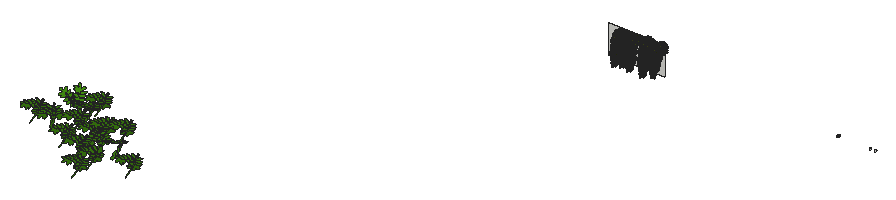
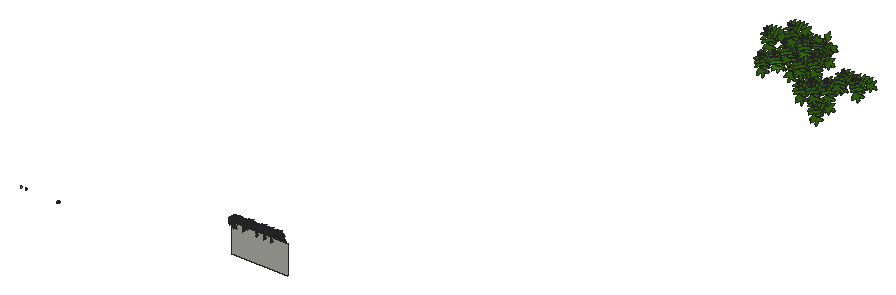
# SketchUp Ruby script. Lengths in inches.
U = 1.inch
M = Sketchup.active_model
def pt(a) = Geom::Point3d.new(a.map { |v| v * U })
def face(e, loops, mat)
  f = e.add_face(loops[0].map { |a| pt(a) })
  loops[1..].each { |l| e.add_face(l.map { |a| pt(a) }).erase! }
  f.material = f.back_material = mat if mat
  f
end
# faces: each face lists its corners as indices into pts; further lists are holes
def faces(e, pts, list, mat = nil) = list.each { |f| face(e, (f[0].is_a?(Array) ? f : [f]).map { |l| l.map { |i| pts[i] } }, mat) }
# xy, xz, yz: faces in a plane at the given z, y or x. An outline is a flat list of corners, or four numbers for a rectangle; further outlines are holes
def ring(l) = l.size == 4 ? [[l[0], l[1]], [l[2], l[1]], [l[2], l[3]], [l[0], l[3]]] : l.each_slice(2).to_a
def flat(e, list, mat, &to3) = list.each { |f| face(e, (f[0].is_a?(Array) ? f : [f]).map { |l| ring(l).map { |u, v| to3.(u, v) } }, mat) }
def xy(e, z, list, mat = nil) = flat(e, list, mat) { |x, y| [x, y, z] }
def xz(e, y, list, mat = nil) = flat(e, list, mat) { |x, z| [x, y, z] }
def yz(e, x, list, mat = nil) = flat(e, list, mat) { |y, z| [x, y, z] }
def lines(e, pts, list) = list.each { |a, b| e.add_line(pt(pts[a]), pt(pts[b])) }
# prism: a flat outline (further loops are holes) pulled along v
def prism(e, loops, v, mat = nil)
  f = face(e, loops, mat); d = Geom::Vector3d.new(v.map { |x| x * U })
  f.pushpull(f.normal.samedirection?(d) ? d.length : -d.length)
end
def box(e, o, s, mat = nil) = prism(e, [[o, [o[0] + s[0], o[1], o[2]], [o[0] + s[0], o[1] + s[1], o[2]], [o[0], o[1] + s[1], o[2]]]], [0, 0, s[2]], mat)
def at(x, y, z, deg = 0) = Geom::Transformation.translation(pt([x, y, z])) * Geom::Transformation.rotation(ORIGIN, Z_AXIS, deg.degrees)
def axes(o, x, y, z) = Geom::Transformation.new([*x, 0, *y, 0, *z, 0, *pt(o).to_a, 1])
def part(name) = M.definitions.add(name)
# library, detail: a bought-in or finely detailed component or shape, given as its bounding box
def library(name, o, s) = part(name).tap { |d| box(d.entities, o, s) }
def detail(e, o, s) = box(e.add_group.entities, o, s)
def put(e, d, t, mat = nil) = e.add_instance(d, t).tap { |i| i.material = mat if mat }
def group(e, t, mat = nil) = e.add_group.tap { |g| g.transformation = t; g.material = mat if mat }.entities
root = M.entities
M.materials.add("asdfasdfasdfasdf").color = [186, 198, 91]
M.materials.add("hojas").color = [70, 150, 19]
M.materials.add("leaf1_smaller_cleanasdfasfasdfas").color = [88, 95, 33]
M.materials.add("leaf2_smaller_cleansadfasdfasdfasd").color = [55, 66, 19]
c1 = part("rama-acacia")
p = [[-13.53,0.69,-1.07],[-13.38,0.86,-0.98],[-13.61,0.85,-1.06],[-14.07,0.85,-1.21],[-15.17,0.86,-1.58],[-15.95,0.92,-1.83],
  [-16.01,1,-1.83],[-16.01,1.17,-1.78],[-16.07,1.93,-1.6],[-16.4,2.73,-1.5],[-16.65,3.06,-1.5],[-17.13,4.01,-1.41],
  [-17.78,4.7,-1.44],[-18.28,5.07,-1.51],[-18.57,5.18,-1.58],[-18.91,5.47,-1.62],[-19.07,5.48,-1.67],[-19.35,5.61,-1.73],
  [-19.51,5.64,-1.78],[-19.38,5.57,-1.75],[-19.33,5.5,-1.75],[-19.31,5.23,-1.82],[-19.38,5.08,-1.89],[-19.41,4.84,-1.96],
  [-19.36,4.59,-2.01],[-19.43,4.55,-2.04],[-19.36,4.15,-2.125],[-19.21,3.7,-2.19],[-18.875,3.1,-2.24],[-18.61,2.78,-2.24],
  [-17.83,2.19,-2.13],[-17.4375,1.85,-2.09],[-17.04,1.49,-2.05],[-16.61,1.24,-1.97],[-16.17,1.0625,-1.87],[-16.06,0.95,-1.86],
  [-16.06,0.91,-1.87],[-16.32,0.9,-1.96],[-16.7,0.88,-2.1],[-17.05,0.91,-2.21],[-17.61,1.15,-2.33],[-18.06,1.29,-2.45],
  [-18.88,1.53,-2.67],[-20.25,1.46,-3.15],[-20.59,1.49,-3.26],[-20.79,1.37,-3.36],[-21.08,1.2,-3.5],[-21.28,1.22,-3.5625],
  [-21.48,0.94,-3.71],[-21.79,0.5,-3.93],[-22.02,0.17,-4.1],[-22.11,0.05,-4.16],[-22.21,-0.02,-4.21],[-22.375,-0.05,-4.28],
  [-22.375,-0.07,-4.28],[-22.18,-0.09,-4.22],[-22.11,-0.07,-4.19],[-21.78,-0.1,-4.09],[-21.6,-0.18,-4.05],[-21.52,-0.27,-4.04],
  [-21.33,-0.33,-4],[-20.94,-0.54,-3.92],[-20.6875,-0.63,-3.86],[-20.54,-0.68,-3.82],[-20.42,-0.67,-3.78],[-20.09,-0.46,-3.61],
  [-19.8,-0.24,-3.45],[-19.21,-0.02,-3.19],[-18.48,0.08,-2.92],[-17.72,0.38,-2.58],[-17.4,0.5,-2.4375],[-16.93,0.75,-2.21],
  [-16.78,0.8,-2.15],[-16.1,0.83,-1.91],[-16.0625,0.81,-1.9],[-16.08,0.77,-1.91],[-16.27,0.72,-1.99],[-16.88,0.39,-2.29],
  [-17.1875,0.15,-2.46],[-17.27,0.02,-2.52],[-17.94,-0.52,-2.89],[-17.94,-0.59,-2.91],[-18.08,-0.68,-2.99],[-18.13,-0.86,-3.05],
  [-18.56,-1.55,-3.38],[-18.71,-2.11,-3.58],[-18.79,-2.61,-3.74],[-18.86,-2.84,-3.83],[-18.87,-3.07,-3.89],[-18.84,-3.22,-3.92],
  [-18.8,-3.26,-3.92],[-18.76,-3.47,-3.96],[-18.76,-3.6,-4],[-18.67,-3.8,-4.02],[-18.61,-3.92,-4.04],[-18.58,-4.11,-4.07],
  [-18.53,-4.18,-4.08],[-18.58,-4.35,-4.14],[-18.65,-4.43,-4.18],[-18.72,-4.51,-4.23],[-18.8125,-4.51,-4.26],[-18.8125,-4.53,-4.26],
  [-18.72,-4.54,-4.24],[-18.66,-4.49,-4.21],[-18.58,-4.43,-4.16],[-18.35,-4.23,-4.03],[-18.32,-4.17,-4],[-18.22,-4.125,-3.95],
  [-18.1,-4,-3.88],[-17.79,-3.72,-3.7],[-17.68,-3.51,-3.61],[-17.32,-3.13,-3.38],[-17.24,-2.94,-3.31],[-16.78,-2.12,-2.93],
  [-16.48,-1.78,-2.73],[-16.3,-1.28,-2.54],[-16.05,-0.75,-2.3125],[-15.89,-0.2,-2.11],[-15.89,0.39,-1.95],[-15.96,0.79,-1.87],
  [-15.91,0.82,-1.84],[-15.27,0.8,-1.63],[-14.18,0.76,-1.27],[-13.78,0.73,-1.15],[-13.78,0.67,-1.16],[-14.23,0.54,-1.35],
  [-14.65,0.33,-1.55],[-14.97,0.02,-1.74],[-15.25,-0.36,-1.9375],[-15.57,-0.72,-2.14],[-15.96,-1.64,-2.52],[-16.2,-2.51,-2.84],
  [-16.2,-3.12,-3],[-16.14,-3.41,-3.06],[-16.1,-3.75,-3.14],[-16.1,-4.09,-3.23],[-16.2,-4.25,-3.3],[-16.2,-4.28,-3.3125],
  [-16.08,-4.19,-3.24],[-15.98,-4.08,-3.18],[-15.96,-3.94,-3.14],[-15.96,-3.8125,-3.1],[-15.9,-3.72,-3.06],[-15.68,-3.55,-2.9375],
  [-15.51,-3.49,-2.86],[-15.3,-3.33,-2.75],[-15.23,-3.17,-2.68],[-15.01,-3.03,-2.57],[-14.875,-2.83,-2.47],[-14.6,-2.59,-2.3125],
  [-14.4,-2.27,-2.16],[-14.12,-1.6,-1.89],[-13.91,-1.1,-1.68],[-13.67,-0.83,-1.53],[-13.53,-0.45,-1.38],[-13.53,0.67,-1.08],
  [-12.41,6.01,0.65],[-12.44,6.14,0.68],[-12.41,6.29,0.73],[-12.43,6.29,0.73],[-12.44,6.26,0.72],[-12.47,6.15,0.68],
  [-12.49,6.07,0.66],[-12.57,5.75,0.55],[-12.67,5.36,0.43],[-12.79,4.875,0.28],[-12.83,4.52,0.18],[-12.83,3.99,0.04],
  [-12.73,3.11,-0.18],[-12.58,2.52,-0.3125],[-12.3,1.97,-0.41],[-11.88,1.51,-0.46],[-11.37,1.0625,-0.48],[-10.75,0.75,-0.45],
  [-10.75,0.68,-0.47],[-12.55,0.7,-0.79],[-13.21,0.79,-0.89],[-13.2,0.67,-0.92],[-12.56,0.62,-0.82],[-11.15,0.56,-0.58],
  [-10.79,0.54,-0.52],[-10.72,0.52,-0.51],[-10.72,0.5,-0.52],[-10.87,0.47,-0.55],[-11.14,0.41,-0.62],[-11.39,0.27,-0.7],
  [-11.625,-0.01,-0.82],[-11.8,-0.43,-0.96],[-11.83,-0.57,-1],[-12.02,-1.08,-1.17],[-12.1,-1.39,-1.27],[-12.17,-1.95,-1.4375],
  [-12.17,-2.77,-1.65],[-12.09,-3.59,-1.86],[-11.86,-4.26,-2],[-11.8125,-4.4,-2.03],[-11.84,-4.49,-2.05],[-11.91,-4.6,-2.1],
  [-11.97,-4.65,-2.12],[-11.98,-4.67,-2.13],[-11.92,-4.65,-2.11],[-11.84,-4.59,-2.08],[-11.77,-4.52,-2.05],[-11.74,-4.47,-2.03],
  [-11.37,-4.3125,-1.92],[-10.95,-4.0625,-1.78],[-10.82,-3.89,-1.71],[-10.64,-3.57,-1.59],[-10.41,-3.05,-1.41],[-10.27,-2.73,-1.3],
  [-10.07,-1.88,-1.03],[-10.15,-0.71,-0.73],[-10.31,-0.1,-0.6],[-10.5,0.4,-0.5],[-10.5,0.48,-0.48],[-10.44,0.53,-0.45],
  [-10.39,0.64,-0.42],[-10.52,0.73,-0.42],[-10.44,0.93,-0.35],[-10.44,1.2,-0.28],[-10.32,1.47,-0.18],[-10.48,2.6875,0.12],
  [-10.43,2.96,0.2],[-10.75,3.87,0.38],[-11.26,4.93,0.57],[-11.8,5.54,0.64],[-12.37,5.93,0.64],[-7.78,0.19,-0.06],
  [-7.78,0.25,-0.04],[-7.75,0.39,0],[-7.89,0.4,-0.02],[-7.96,0.46,-0.02],[-7.96,0.49,-0.01],[-7.76,0.62,0.06],
  [-7.53,0.99,0.2],[-7.31,1.78,0.45],[-7.31,2.74,0.71],[-7.63,3.6875,0.9],[-8.02,4.57,1.07],[-8.66,5.23,1.13],
  [-8.83,5.4,1.14],[-8.92,5.54,1.16],[-9.1,5.64,1.16],[-9.08,5.6,1.15],[-9.02,5.56,1.15],[-8.94,5.46,1.14],
  [-8.9,5.37,1.12],[-8.9375,5.25,1.08],[-9.14,4.92,0.96],[-9.31,4.5625,0.83],[-9.39,3.73,0.6],[-9.44,2.76,0.32],
  [-9.23,1.59,0.05],[-8.82,0.9,-0.06],[-8.36,0.59,-0.0625],[-8.14,0.51,-0.04],[-8.05,0.48,-0.03],[-8.05,0.46,-0.04],
  [-8.12,0.43,-0.06],[-10.1,0.49,-0.4],[-8.22,0.3125,-0.11],[-8.22,0.25,-0.125],[-8.53,0.13,-0.21],[-8.8,-0.16,-0.34],
  [-8.96,-0.61,-0.49],[-8.96,-0.87,-0.56],[-9.16,-1.42,-0.74],[-9.13,-1.77,-0.83],[-9.09,-1.83,-0.84],[-9.125,-1.92,-0.87],
  [-9.125,-2.13,-0.93],[-9.08,-2.23,-0.95],[-9.15,-2.39,-1],[-9.11,-2.67,-1.07],[-9.03,-2.86,-1.11],[-9.07,-3.03,-1.16],
  [-8.97,-3.23,-1.19],[-8.93,-3.44,-1.24],[-8.93,-3.71,-1.32],[-8.79,-4.05,-1.38],[-8.7,-4.25,-1.42],[-8.7,-4.39,-1.46],
  [-8.76,-4.53,-1.5],[-8.77,-4.65,-1.54],[-8.64,-4.55,-1.49],[-8.27,-4.22,-1.33],[-8.1875,-4.06,-1.27],[-8.07,-3.98,-1.23],
  [-7.98,-3.79,-1.17],[-7.79,-3.59,-1.08],[-7.64,-3.3,-0.97],[-7.64,-3.25,-0.96],[-7.59,-3.21,-0.9375],[-7.52,-2.93,-0.85],
  [-7.52,-2.85,-0.83],[-7.47,-2.81,-0.81],[-7.3,-2.09,-0.59],[-7.32,-2.01,-0.57],[-7.27,-1.95,-0.54],[-7.1875,-1.57,-0.42],
  [-7.17,-1.46,-0.39],[-7.17,-1.16,-0.3125],[-7.23,-0.61,-0.17],[-7.49,-0.15,-0.1],[-13.39,-0.07,-1.23],[-13.39,0.25,-1.14],
  [-13.49,0.5625,-1.09],[-13.8,1.01,-1.08],[-13.61,0.91,-1.04],[-13.38,0.92,-0.96],[-13.32,1.03,-0.91],[-13.32,1.35,-0.82],
  [-13.28,1.49,-0.77],[-13.28,1.99,-0.64],[-13.44,2.67,-0.51],[-13.72,3.31,-0.43],[-13.93,3.71,-0.4],[-14.1,4.39,-0.27],
  [-14.5625,5.06,-0.25],[-14.89,5.62,-0.21],[-15.33,6.1,-0.23],[-15.65,6.8,-0.15],[-15.79,6.89,-0.18],[-15.61,6.52,-0.22],
  [-15.51,6.32,-0.24],[-15.45,6.28,-0.23],[-15.52,6,-0.32],[-15.63,5.6875,-0.45],[-15.77,4.97,-0.68],[-15.7,4.25,-0.85],
  [-15.46,3,-1.11],[-15,2.03,-1.21],[-14.3,1.29,-1.17],[-4.5625,0.33,0.09],[-4.22,0.49,0.13],[-4,0.7,0.1875],
  [-3.86,0.99,0.26],[-3.77,1.41,0.38],[-3.7,1.73,0.46],[-3.77,1.99,0.53],[-3.85,2.17,0.58],[-3.88,2.57,0.6875],
  [-3.98,2.9,0.78],[-4.0625,2.97,0.8],[-4.1,3.14,0.84],[-4.1875,3.25,0.87],[-4.27,3.55,0.95],[-4.31,3.71,0.99],
  [-4.42,3.9,1.04],[-4.625,4.2,1.125],[-4.72,4.39,1.18],[-4.89,4.57,1.23],[-4.98,4.73,1.27],[-5,4.72,1.26],
  [-5.01,4.51,1.21],[-4.96,4.32,1.16],[-4.97,4.27,1.14],[-5.14,3.78,1.01],[-5.3,3.39,0.91],[-5.44,2.76,0.74],
  [-5.5,2.09,0.56],[-5.57,1.78,0.48],[-5.57,1.42,0.38],[-5.57,1.09,0.29],[-5.47,0.72,0.19],[-5.22,0.44,0.12],
  [-4.93,0.27,0.07],[-4.76,0.22,0.06],[-4.76,0.18,0.05],[-4.83,0.16,0.04],[-5.26,0,0],[-5.34,-0.04,-0.01],
  [-5.47,-0.22,-0.06],[-5.51,-0.6,-0.16],[-5.42,-1.09,-0.29],[-5.28,-1.49,-0.4],[-5.21,-1.87,-0.5],[-5.11,-2.15,-0.57],
  [-5.08,-2.34,-0.63],[-5.01,-2.47,-0.66],[-4.96,-2.69,-0.72],[-4.86,-2.9375,-0.79],[-4.84,-3.07,-0.82],[-4.77,-3.18,-0.85],
  [-4.74,-3.43,-0.92],[-4.7,-3.71,-0.99],[-4.62,-3.89,-1.04],[-4.58,-3.98,-1.07],[-4.58,-3.83,-1.03],[-4.51,-3.67,-0.98],
  [-4.3,-3.32,-0.89],[-4.16,-3.09,-0.83],[-4.16,-2.98,-0.8],[-4.11,-2.92,-0.78],[-4.02,-2.8,-0.75],[-3.95,-2.59,-0.69],
  [-3.95,-2.33,-0.625],[-3.86,-2.26,-0.6],[-3.86,-2.02,-0.54],[-3.86,-1.44,-0.39],[-3.94,-1.22,-0.33],[-3.94,-1.08,-0.29],
  [-4,-0.96,-0.26],[-4,-0.87,-0.23],[-4.0625,-0.8125,-0.22],[-4.16,-0.54,-0.14],[-4.39,-0.24,-0.06],[-4.61,-0.08,-0.02],
  [-4.77,-0.03,-0.01],[-4.77,-0.01,0],[-4.65,-0.01,0],[-4.61,0.19,0.05],[-4.66,0.23,0.0625],[-4.63,0.29,0.08],
  [-4.07,0.17,0.04],[0,-0.24,-0.06],[0,0,0],[-0.5,0.04,0.01],[-1.58,0.08,0.02],[-13.78,0.67,-1.08]]
faces(c1.entities,p,[[0,1,2,3,4,5,6,7,8,9,10,11,12,13,14,15,16,17,18,19,20,21,22,23,24,25,26,27,28,29,30,31,32,33,34,35,36,37,38,39,40,41,42,43,44,45,46,47,48,49,50,51,52,53,54,55,56,57,58,59,60,61,62,63,64,65,66,67,68,69,70,71,72,73,74,75,76,77,78,79,80,81,82,83,84,85,86,87,88,89,90,91,92,93,94,95,96,97,98,99,100,101,102,103,104,105,106,107,108,109,110,111,112,113,114,115,116,117,118,119,120,121,122,123,124,125,126,127,128,129,130,131,132,133,134,135,136,137,138,139,140,141,142,143,144,145,146,147,148,149,150,151,152,153,154,155],[156,157,158,159,160,161,162,163,164,165,166,167,168,169,170,171,172,173,174,175,176,177,178,179,180,181,182,183,184,185,186,187,188,189,190,191,192,193,194,195,196,197,198,199,200,201,202,203,204,205,206,207,208,209,210,211,212,213,214,215,216,217,218,219,220,221,222,223,224,225,226],[227,228,229,230,231,232,233,234,235,236,237,238,239,240,241,242,243,244,245,246,247,248,249,250,251,252,253,254,255,256,257,258,216,215,259,260,261,262,263,264,265,266,267,268,269,270,271,272,273,274,275,276,277,278,279,280,281,282,283,284,285,286,287,288,289,290,291,292,293,294,295,296,297,298,299,300,301,302,303],[154,304,305,306,155],[307,308,1,309,310,311,312,313,314,315,316,317,318,319,320,321,322,323,324,325,326,327,328,329,330,331,332],[333,334,335,336,337,338,339,340,341,342,343,344,345,346,347,348,349,350,351,352,353,354,355,356,357,358,359,360,361,362,363,364,365,366,367,368,369,370,371,372,373,374,375,376,377,378,379,380,381,382,383,384,385,386,387,388,389,390,391,392,393,394,395,396,397,398,399,400,401,402,403,404,405,406,407,408,409,410,411,412,413],[0,177,1],[308,2,1],
  [176,1,177],[414,411,410,415,416,417,418],[228,370,229],[369,229,370]],"hojas")
lines(c1.entities,p,[[155,419]])
c2 = part("Group\#150")
put(c2.entities,c1,axes([10.13,10.27,0],[0.45315,0.21131,0],[-0.21131,0.45315,0],[0,0,0.5]))
put(c2.entities,c1,axes([10.13,10.27,0],[0.11638,0.47539,0.10227],[-0.48087,0.12813,-0.0484],[-0.07223,-0.08709,0.48703]))
put(c2.entities,c1,axes([9.58,10.26,-0.7],[0.1449,0.38901,-0.2787],[-0.10883,0.31035,0.37662],[0.46601,-0.04848,0.17461]))
c3 = part("Group\#151")
put(c3.entities,c2,axes([24.99,4.24,9.59],[0.78856,0.61496,0],[0.01473,-0.01889,0.99971],[0.61478,-0.78833,-0.02396]))
put(c3.entities,c2,axes([39.5,6.625,12.55],[0.6544,0.49291,0.57341],[-0.44023,-0.3682,0.81892],[0.61478,-0.78833,-0.02396]))
put(c3.entities,c2,axes([32.34,3.7,6.88],[0.78856,0.61496,0],[0.01473,-0.01889,0.99971],[0.61478,-0.78833,-0.02396]))
put(c3.entities,c2,axes([43.14,6.65,17.54],[0.78856,0.61496,0],[0.35273,-0.4523,0.81915],[0.50374,-0.64595,-0.57358]))
put(c3.entities,c2,axes([12.2,6.2,16.68],[0.7209,0.54936,0.4225],[-0.31991,-0.27701,0.90605],[0.61478,-0.78833,-0.02396]))
put(c3.entities,c2,axes([49.9375,3.79,26.09],[0.78856,0.61496,0],[0.01473,-0.01889,0.99971],[0.61478,-0.78833,-0.02396]))
put(c3.entities,c2,axes([36.11,4.9375,33.94],[0.78856,0.61496,0],[0.01473,-0.01889,0.99971],[0.61478,-0.78833,-0.02396]))
put(c3.entities,c2,axes([39.61,3.79,23.47],[0.78856,0.61496,0],[0.01473,-0.01889,0.99971],[0.61478,-0.78833,-0.02396]))
put(c3.entities,c2,axes([25.59,6.5625,46.47],[-0.40704,-0.29112,-0.86578],[0.67555,0.54201,-0.49986],[0.61478,-0.78833,-0.02396]))
put(c3.entities,c2,axes([54.97,1.98,11.65],[0.78856,0.61496,0],[0.01473,-0.01889,0.99971],[0.61478,-0.78833,-0.02396]))
put(c3.entities,c2,axes([32.97,3.79,19.14],[0.78856,0.61496,0],[0.01473,-0.01889,0.99971],[0.61478,-0.78833,-0.02396]))
put(c3.entities,c2,axes([24.24,3.79,21.99],[0.78856,0.61496,0],[0.01473,-0.01889,0.99971],[0.61478,-0.78833,-0.02396]))
put(c3.entities,c2,axes([16.86,4.24,12.3],[0.78856,0.61496,0],[0.01473,-0.01889,0.99971],[0.61478,-0.78833,-0.02396]))
put(c3.entities,c2,axes([1.23,3.9375,19.07],[0.78856,0.61496,0],[0.01473,-0.01889,0.99971],[0.61478,-0.78833,-0.02396]))
put(c3.entities,c2,axes([29.05,5.25,29.11],[0.78856,0.61496,0],[0.21033,-0.2697,0.93969],[0.57787,-0.741,-0.34202]))
put(c3.entities,c2,axes([24.16,3.79,-0.1],[0.78856,0.61496,0],[0.01473,-0.01889,0.99971],[0.61478,-0.78833,-0.02396]))
c4 = part("leaf1a")
p = [[1.06,3.74,11.78],[8.28,8.7,-0.64],[9.51,5.4,26.1],[17.76,4.04,11.26],[17.85,2.23,20],[14.31,3.29,26.73],
  [3.78,3.8125,25.98],[-0.21,2.38,19.72]]
faces(c4.entities,p,[[0,1,2],[2,1,3],[3,4,5],[3,5,2],[6,7,0],[0,2,6]],"leaf1_smaller_cleanasdfasfasdfas")
c5 = part("leaf2a")
p = [[1.4375,3.56,10.81],[8.71,6.8,-0.73],[9.51,3.5,26.59],[16.66,3.91,9.8],[17.86,1.3,19.21],[14.9,1.58,24.92],
  [5.15,2.55,24.01],[1.29,1.87,19.875]]
faces(c5.entities,p,[[0,1,2],[2,1,3],[3,4,5],[3,5,2],[6,7,0],[0,2,6]],"leaf2_smaller_cleansadfasdfasdfasd")
c6 = part("Group\#220")
put(c6.entities,c5,axes([6.68,1.92,2.42],[-0.04671,0.11082,0.08136],[0.07715,0.09226,-0.08136],[-0.11379,0.01705,-0.08856]))
put(c6.entities,c4,axes([1.26,0.54,1.25],[0.13756,-0.04533,0.01029],[0.0079,-0.00888,-0.14471],[0.04581,0.13766,-0.00594]))
put(c6.entities,c5,axes([-0.51,4.89,1.49],[-0.00057,-0.14139,-0.03304],[0.00922,0.03294,-0.14111],[0.14491,-0.00265,0.00885]))
put(c6.entities,c4,axes([4.37,7.98,1.26],[-0.14226,-0.02905,0],[0,0,-0.1452],[0.02905,-0.14226,0]))
put(c6.entities,c4,axes([1.46,4.03,4.07],[0.06242,-0.12847,-0.02614],[-0.10319,-0.03029,-0.09755],[0.08086,0.06051,-0.10432]))
c7 = part("leaf_a")
p = [[1.43,4.41,0.74],[1.39,4.36,0.69],[1.39,4.61,0.21],[1.43,4.67,0.24],[1.35,4.41,0.74],[1.35,4.67,0.24],
  [1.35,3.9,1.02],[1.43,3.9,1.02],[1.39,3.89,0.95],[1.39,3.35,0.9],[1.43,3.34,0.96],[1.35,3.34,0.96]]
faces(c7.entities,p,[[0,1,2,3],[1,4,5,2],[4,0,3,5],[3,2,5],[6,7,0,4],[8,6,4,1],[7,8,1,0],[9,10,11],
  [9,11,6,8],[10,9,8,7],[11,10,7,6]],"asdfasdfasdfasdf")
put(c7.entities,c5,axes([0,-0.08,0.875],[0.1452,0,0],[0,0.02746,-0.14258],[0,0.14258,0.02746]))
c8 = part("leaf_b")
prism(c8.entities,[[[1.36,4.21,-0.25],[1.31,4.13,-0.29],[1.26,4.21,-0.25]]],[0,-0.66,1.14],"asdfasdfasdfasdf")
put(c8.entities,c4,axes([0,-0.1,0.68],[0.1452,-0.0002,0],[0.00006,0.04124,-0.13922],[0.00019,0.13922,0.04124]))
c9 = part("Group\#209")
p = [[2.87,4.13,4.15],[2.98,3.98,4.12],[2.98,4.66,2.59],[2.87,4.8,2.65],[3.09,4.13,4.15],[3.09,4.8,2.65],
  [2.87,4.13,6.07],[2.98,3.98,6.12],[3.09,4.13,6.07],[2.87,5.04,7.34],[2.98,4.91,7.43],[3.09,5.04,7.34]]
faces(c9.entities,p,[[0,1,2,3],[1,4,5,2],[6,7,1,0],[7,8,4,1],[9,10,7,6],[10,11,8,7]],"asdfasdfasdfasdf")
put(c9.entities,c7,axes([0.86,0.51,1.53],[0.95176,-0.27809,0.12967],[0.18405,0.85554,0.48392],[-0.24551,-0.43671,0.86545]))
put(c9.entities,c8,axes([-0.97,2.96,6.52],[0.70711,-0.61237,-0.35355],[0.70711,0.61237,0.35355],[0,-0.5,0.86603]))
put(c9.entities,c7,axes([3.23,0.39,0.41],[0.82736,0.50176,-0.25242],[-0.32519,0.79434,0.5131],[0.45796,-0.34244,0.82037]))
put(c9.entities,c7,axes([3.25,-0.58,4.78],[0.8251,0.44069,-0.35355],[-0.31829,0.8796,0.35355],[0.46679,-0.17918,0.86603]))
c10 = part("Group\#2")
p = [[1.22,4.71,2.14],[1.31,4.57,2.14],[2.16,4.71,3.79],[2.24,4.57,3.77],[1.39,4.71,2.14],[2.33,4.71,3.79],
  [1.93,3.51,6.2],[1.85,3.64,6.23],[2.02,3.64,6.23],[0.93,3.38,8.58],[0.85,3.52,8.58],[1.02,3.52,8.58],
  [0.81,3.57,10.77],[0.72,3.71,10.73],[0.89,3.71,10.73],[1.31,4.57,13.2],[1.22,4.7,13.15],[1.39,4.7,13.15]]
faces(c10.entities,p,[[0,1,2],[3,2,1],[1,4,3],[5,3,4],[6,7,3],[6,3,8],[2,3,7],[5,8,3],
  [9,10,6],[9,6,11],[7,6,10],[8,11,6],[9,11,12],[9,12,10],[13,10,12],[14,12,11],
  [12,15,13],[12,14,15],[16,13,15],[17,15,14]],"asdfasdfasdfasdf")
put(c10.entities,c8,axes([3.93,1.17,1.97],[0.75139,0.49793,0.43299],[-0.65983,0.56085,0.50006],[0.00615,-0.66145,0.74997]))
put(c10.entities,c8,axes([6.23,5.09,1.92],[-0.36585,0.92196,0.12706],[-0.79398,-0.38042,0.47421],[0.48554,0.0726,0.87119]))
put(c10.entities,c8,axes([0.03,0.92,11.26],[1,0,0],[0,0.86603,0.5],[0,-0.5,0.86603]))
put(c10.entities,c7,axes([4.37,2.0625,9.11],[0.45529,0.76896,0.44879],[-0.86129,0.25267,0.44084],[0.22559,-0.58725,0.77733]))
put(c10.entities,c7,axes([1.89,-0.25,4.42],[0.88717,0.14116,0.43931],[-0.36372,0.79981,0.47751],[-0.28396,-0.58342,0.76091]))
put(c10.entities,c7,axes([-0.4,-0.0625,7.9],[0.80178,0.42258,-0.42258],[0,0.70711,0.70711],[0.59763,-0.56694,0.56694]))
put(c10.entities,c8,axes([0.05,0.6875,0.65],[0.97178,0.10445,-0.21151],[0.0126,0.87237,0.48869],[0.23556,-0.47756,0.84643]))
put(c10.entities,c7,axes([5.56,1.19,4.08],[0.24789,0.96746,-0.05068],[-0.86286,0.24427,0.4425],[0.44048,-0.06596,0.89533]))
put(c10.entities,c8,axes([4.91,2.14,7.29],[-0.04249,0.96546,-0.25705],[-0.89911,0.07524,0.4312],[0.43565,0.24944,0.86486]))
c11 = part("Group\#208")
put(c11.entities,c5,axes([5.59,5.52,3.3],[-0.07606,0.12201,-0.02028],[0.09645,0.0436,-0.0994],[-0.07744,-0.06554,-0.10388]))
put(c11.entities,c5,axes([7.69,4.27,1.08],[-0.09839,0.10661,0.00609],[-0.00698,0.00184,-0.14502],[-0.10656,-0.09856,0.00388]))
put(c11.entities,c4,axes([3.51,6.9,2.1],[-0.1403,-0.03711,-0.00465],[-0.00046,0.01976,-0.14385],[0.03739,-0.13898,-0.01921]))
put(c11.entities,c5,axes([2.18,0.07,1.375],[0.14025,0.00096,-0.03757],[-0.03758,0.00358,-0.14021],[0,0.14515,0.00371]))
put(c11.entities,c4,axes([-0.62,2,1.16],[0.081,-0.0806,-0.00996],[0.00004,0.01411,-0.11384],[0.08122,0.08039,0.00999]))
c12 = part("Group\#221")
p = [[1.22,4.71,2.14],[1.31,4.57,2.14],[2.16,4.71,3.79],[2.24,4.57,3.77],[1.39,4.71,2.14],[2.33,4.71,3.79],
  [1.93,3.51,6.2],[1.85,3.64,6.23],[2.02,3.64,6.23],[0.93,3.38,8.58],[0.85,3.52,8.58],[1.02,3.52,8.58],
  [0.81,3.57,10.77],[0.72,3.71,10.73],[0.89,3.71,10.73],[1.31,4.57,13.2],[1.22,4.7,13.15],[1.39,4.7,13.15]]
faces(c12.entities,p,[[0,1,2],[3,2,1],[1,4,3],[5,3,4],[6,7,3],[6,3,8],[2,3,7],[5,8,3],
  [9,10,6],[9,6,11],[7,6,10],[8,11,6],[9,11,12],[9,12,10],[13,10,12],[14,12,11],
  [12,15,13],[12,14,15],[16,13,15],[17,15,14]],"asdfasdfasdfasdf")
put(c12.entities,c8,axes([3.93,1.17,1.97],[0.75139,0.49793,0.43299],[-0.65983,0.56085,0.50006],[0.00615,-0.66145,0.74997]))
put(c12.entities,c8,axes([6.23,5.09,1.92],[-0.36585,0.92196,0.12706],[-0.79398,-0.38042,0.47421],[0.48554,0.0726,0.87119]))
put(c12.entities,c8,axes([0.03,0.92,11.26],[1,0,0],[0,0.86603,0.5],[0,-0.5,0.86603]))
put(c12.entities,c7,axes([4.37,2.0625,9.11],[0.45529,0.76896,0.44879],[-0.86129,0.25267,0.44084],[0.22559,-0.58725,0.77733]))
put(c12.entities,c7,axes([1.89,-0.25,4.42],[0.88717,0.14116,0.43931],[-0.36372,0.79981,0.47751],[-0.28396,-0.58342,0.76091]))
put(c12.entities,c7,axes([-0.4,-0.0625,7.9],[0.80178,0.42258,-0.42258],[0,0.70711,0.70711],[0.59763,-0.56694,0.56694]))
put(c12.entities,c8,axes([0.05,0.6875,0.65],[0.97178,0.10445,-0.21151],[0.0126,0.87237,0.48869],[0.23556,-0.47756,0.84643]))
put(c12.entities,c7,axes([5.56,1.19,4.08],[0.24789,0.96746,-0.05068],[-0.86286,0.24427,0.4425],[0.44048,-0.06596,0.89533]))
put(c12.entities,c8,axes([4.91,2.14,7.29],[-0.04249,0.96546,-0.25705],[-0.89911,0.07524,0.4312],[0.43565,0.24944,0.86486]))
c13 = part("Trailing philodendron")
put(c13.entities,c4,axes([3.65,12.52,19.68],[-0.0527,-0.13492,0.0101],[-0.03487,0.00307,-0.14092],[0.13073,-0.05357,-0.03351]))
put(c13.entities,c4,axes([5.13,11.34,20.6],[-0.03432,-0.12484,0.06572],[-0.08608,-0.03507,-0.11155],[0.11179,-0.06533,-0.06572]))
put(c13.entities,c5,axes([2.61,13.04,18.63],[0.05838,-0.12752,0.03758],[0.01564,-0.03417,-0.14025],[0.13202,0.06044,0]))
put(c13.entities,c5,axes([3.7,9.83,20.73],[-0.00129,-0.14519,0],[-0.0726,0.00064,-0.12575],[0.12574,-0.00112,-0.0726]))
put(c13.entities,c5,axes([11.375,11.11,20.23],[-0.14171,0.00126,0.03163],[-0.02867,0.05638,-0.1307],[-0.01341,-0.1338,-0.05478]))
put(c13.entities,c4,axes([2.4375,12.45,15.12],[-0.02375,-0.14324,0],[0.13106,-0.02173,-0.05859],[0.05781,-0.00958,0.13285]))
put(c13.entities,c4,axes([9.62,10.68,22.01],[0.05693,0.12487,-0.04742],[0.05061,-0.06787,-0.11796],[-0.12361,0.02972,-0.07014]))
put(c13.entities,c4,axes([11.63,16.35,20.5625],[-0.12691,-0.00762,0.07014],[-0.06947,0.03872,-0.12148],[-0.01233,-0.13973,-0.03749]))
put(c13.entities,c4,axes([12.51,17.52,17.81],[-0.1445,0.01001,0.0102],[-0.01383,-0.07182,-0.12544],[-0.0036,-0.1258,0.07242]))
put(c13.entities,c5,axes([9.09,6.34,22.72],[-0.09269,-0.05068,-0.09962],[-0.03661,0.13604,-0.03515],[0.1056,0.00268,-0.09962]))
put(c13.entities,c4,axes([4.83,12.62,22.54],[0.10783,0.09684,-0.00888],[0.09716,-0.10783,0.00397],[-0.00394,-0.00889,-0.14487]))
put(c13.entities,c4,axes([4.94,9.48,20.375],[0.01323,0.07633,0.07653],[0.10803,-0.00667,-0.01203],[-0.00375,0.07738,-0.07653]))
put(c13.entities,c5,axes([14,13.64,21.84],[-0.01852,-0.13907,0.03741],[-0.14373,0.01547,-0.01367],[0.00911,-0.03878,-0.13963]))
put(c13.entities,c5,axes([9.23,4.15,18.71],[0.14198,0.00177,-0.03038],[-0.02867,0.05638,-0.1307],[0.01021,0.13379,0.05548]))
put(c13.entities,c5,axes([5.82,4.5625,15.3],[0.13095,-0.05433,0.03137],[0.06268,0.11013,-0.07089],[0.00273,0.07747,0.12278]))
put(c13.entities,c6,axes([6.59,5.29,16.06],[1.23201,0.26412,0],[-0.26412,1.23201,0],[0,0,1.26]))
put(c13.entities,c9,axes([12.21,1.69,0.66],[-0.82914,0.03045,-0.02227],[0.02366,0.80139,0.21474],[-0.02938,-0.21389,0.80143]))
put(c13.entities,c10,axes([6.8125,1.15,7.57],[0.74375,-0.41052,0.02847],[0.41052,0.73612,-0.11],[0.02847,0.11,0.84237]))
put(c13.entities,c9,axes([-1.68,6.875,13.2],[0.5,-0.86603,0],[0.81585,0.47103,-0.33545],[0.29051,0.16773,0.94206]))
put(c13.entities,c9,axes([1.86,19.56,12.8125],[0.88164,0.4704,0.03781],[0.46333,-0.8476,-0.25863],[0.08962,-0.24554,0.96524]))
g1 = group(c13.entities,at(9.13,11.13,20.67))
put(g1,c5,axes([7.36,4.03,-0.3],[-0.05057,0.11966,-0.06487],[0.07036,-0.03625,-0.12173],[-0.11651,-0.07383,-0.04536]))
put(g1,c5,axes([8.4,1.56,-2.35],[-0.06703,0.12496,-0.03122],[-0.04831,-0.05702,-0.12449],[-0.1194,-0.04708,0.0679]))
put(g1,c4,axes([5.37,5.58,-2.1],[-0.14013,0.0124,0.03596],[-0.03803,-0.04347,-0.13322],[-0.00061,-0.13798,0.0452]))
put(g1,c5,axes([2.45,-0.07,0.8],[0.12002,-0.06072,-0.05468],[-0.07506,-0.04353,-0.11642],[0.03229,0.1245,-0.06737]))
put(g1,c4,axes([0.19,2.38,0.125],[0.05529,-0.09889,0.01797],[-0.03005,-0.03583,-0.10474],[0.09591,0.04578,-0.04318]))
put(c13.entities,c11,axes([17.33,10.54,16.15],[-0.62797,0.46654,0.62289],[-0.59637,-0.80271,0],[0.5,-0.37147,0.78231]))
put(c13.entities,c6,axes([3.44,11.88,17.73],[0.78616,-0.36326,0.5],[0.52263,0.82256,-0.22414],[-0.32986,0.43753,0.83652]))
put(c13.entities,c11,axes([5.5,5.07,16.54],[0.96593,-0.11102,0.2338],[0,0.90334,0.42894],[-0.25882,-0.41432,0.87255]))
put(c13.entities,c9,axes([18.84,3.62,12.91],[-0.80696,-0.59061,0],[-0.57048,0.77946,-0.25882],[-0.15286,0.20886,0.96593]))
put(c13.entities,c10,axes([3.89,0.96,5.21],[0.83948,0.00528,-0.02906],[-0.009,0.83292,-0.10846],[0.02813,0.1087,0.83246]))
put(c13.entities,c10,axes([6.1,0.84,-5.33],[0.875,-0.48296,0.03349],[0.48296,0.86603,-0.12941],[0.03349,0.12941,0.99103]))
put(c13.entities,c10,axes([3.87,-0.55,-8.84],[0.99938,0.00629,-0.0346],[-0.01071,0.99157,-0.12912],[0.03349,0.12941,0.99103]))
put(c13.entities,c9,axes([0.46,6.875,13.01],[0.5,-0.86603,0],[0.81585,0.47103,-0.33545],[0.29051,0.16773,0.94206]))
put(c13.entities,c10,axes([10.39,0.84,1.73],[0.875,-0.48296,0.03349],[0.48296,0.86603,-0.12941],[0.03349,0.12941,0.99103]))
put(c13.entities,c10,axes([-0.75,1.13,2.67],[0.7525,-0.41535,0.0288],[0.41535,0.74478,-0.11129],[0.0288,0.11129,0.85228]))
put(c13.entities,c10,axes([0.04,-0.97,-8.67],[0.735,-0.40569,0.02813],[0.40569,0.72746,-0.1087],[0.02813,0.1087,0.83246]))
put(c13.entities,c10,axes([0.09,-0.6,-7.42],[0.47403,-0.32078,-0.33698],[0.20171,0.57521,-0.26383],[0.41925,0.08595,0.50794]))
put(c13.entities,c10,axes([10.35,0.97,-6.0625],[0.76125,-0.42018,0.02914],[0.42018,0.75344,-0.11259],[0.02914,0.11259,0.86219]))
put(c13.entities,c10,axes([10.78,-1.55,-11.77],[0.72777,-0.42018,0.22517],[0.435,0.75344,0],[-0.19501,0.11259,0.84036]))
put(c13.entities,c10,axes([5.78,-1.55,-20.23],[0.76125,-0.42018,0.02914],[0.42018,0.75344,-0.11259],[0.02914,0.11259,0.86219]))
put(c13.entities,c10,axes([8.72,-1.43,-13.97],[0.65467,-0.36135,0.02506],[0.36135,0.64796,-0.09682],[0.02506,0.09682,0.74149]))
put(c13.entities,c12,axes([1.53,-0.97,-19.86],[0.735,-0.40569,0.02813],[0.40569,0.72746,-0.1087],[0.02813,0.1087,0.83246]))
put(c13.entities,c12,axes([6.23,-2.02,-7.18],[0.55125,-0.30427,0.0211],[0.39555,0.70927,-0.10599],[0.0211,0.08153,0.62435]))
put(c13.entities,c12,axes([6.43,-1.89,6.18],[0.735,-0.40569,0.02813],[0.5274,0.9457,-0.14132],[0.02813,0.1087,0.83246]))
put(c13.entities,c12,axes([10.24,1.09,9.64],[0.62475,-0.34484,0.02391],[0.44829,0.80384,-0.12012],[0.02391,0.0924,0.70759]))
put(c13.entities,c9,axes([1.56,7.74,12.8125],[-0.22619,0.97335,0.03781],[0.93864,0.22817,-0.25863],[0.26037,0.02301,0.96524]))
put(c13.entities,c9,axes([0.65,14.36,12.8125],[0.30411,0.95189,0.03781],[0.92309,-0.28464,-0.25863],[0.23543,-0.11355,0.96524]))
put(c13.entities,c9,axes([7.75,10.38,12.8125],[-0.84074,0.54011,0.03781],[0.51385,0.81797,-0.25863],[0.17062,0.19802,0.96524]))
put(c13.entities,c9,axes([12.92,19.16,12.8125],[0.9234,-0.38197,0.03781],[-0.36017,-0.89632,-0.25863],[-0.13268,-0.22521,0.96524]))
put(c13.entities,c9,axes([6.55,17.22,12.8125],[0.7985,0.60081,0.03781],[0.58857,-0.76596,-0.25863],[0.12643,-0.22877,0.96524]))
put(c13.entities,c9,axes([16.24,8.94,12.8125],[-0.64953,-0.75939,0.03781],[-0.7404,0.62041,-0.25863],[-0.17295,0.19599,0.96524]))
put(c13.entities,c9,axes([15.6875,15.74,12.8125],[0.12972,-0.99083,0.03781],[-0.95648,-0.13509,-0.25863],[-0.26137,0.00261,0.96524]))
put(c13.entities,c9,axes([19.85,8,15.61],[-0.64953,-0.75939,0.03781],[-0.7404,0.62041,-0.25863],[-0.17295,0.19599,0.96524]))
put(c13.entities,c9,axes([18.86,17.5,12.8125],[0.62831,-0.77705,0.03781],[-0.74495,-0.61494,-0.25863],[-0.22422,-0.13434,0.96524]))
put(c13.entities,c9,axes([-0.43,13.28,13.2],[-0.41945,-0.90778,0],[0.85518,-0.39515,-0.33545],[0.30452,-0.14071,0.94206]))
put(c13.entities,c12,axes([4.5625,-2.01,7.45],[0.56595,-0.31238,0.02166],[0.40609,0.72819,-0.10881],[0.02166,0.0837,0.641]))
put(c13.entities,c12,axes([4.48,-2.02,-24.24],[0.55125,-0.30427,0.0211],[0.39555,0.70927,-0.10599],[0.0211,0.08153,0.62435]))
put(c13.entities,c12,axes([4.9,-4.23,-11.04],[0.55125,-0.30427,0.0211],[0.39555,0.70927,-0.10599],[0.0211,0.08153,0.62435]))
put(c13.entities,c11,axes([17.33,10.54,17.41],[-0.62797,0.46654,0.62289],[-0.59637,-0.80271,0],[0.5,-0.37147,0.78231]))
put(c13.entities,c9,axes([-0.03,6.82,20.63],[0.44714,-0.87214,-0.19857],[0.53417,0.43844,-0.7228],[0.71744,0.21712,0.66191]))
put(c13.entities,c9,axes([20.82,12.8,12.8125],[0.12972,-0.99083,0.03781],[-0.95648,-0.13509,-0.25863],[-0.26137,0.00261,0.96524]))
xz(root,776.37,[[3153.83,138.1875,3240.72,183.3125]])
xz(root,799.91,[[3492.44,131.88,3492.73,131.92,3493,132.03,3493.24,132.21,3493.41,132.44,3493.53,132.71,3493.57,133,3493.53,133.29,3493.41,133.57,3493.24,133.8,3493,133.98,3492.73,134.09,3492.44,134.13,3492.15,134.09,3491.88,133.98,3491.65,133.8,3491.47,133.57,3491.35,133.29,3491.32,133,3491.35,132.71,3491.47,132.44,3491.65,132.21,3491.88,132.03,3492.15,131.92],[3543.57,131.88,3543.86,131.92,3544.13,132.03,3544.36,132.21,3544.54,132.44,3544.65,132.71,3544.69,133,3544.65,133.29,3544.54,133.57,3544.36,133.8,3544.13,133.98,3543.86,134.09,3543.57,134.13,3543.27,134.09,3543,133.98,3542.77,133.8,3542.59,133.57,3542.48,133.29,3542.44,133,3542.48,132.71,3542.59,132.44,3542.77,132.21,3543,132.03,3543.27,131.92],[3551.43,131.88,3551.72,131.92,3551.99,132.03,3552.22,132.21,3552.4,132.44,3552.52,132.71,3552.55,133,3552.52,133.29,3552.4,133.57,3552.22,133.8,3551.99,133.98,3551.72,134.09,3551.43,134.13,3551.14,134.09,3550.87,133.98,3550.63,133.8,3550.45,133.57,3550.34,133.29,3550.3,133,3550.34,132.71,3550.45,132.44,3550.63,132.21,3550.87,132.03,3551.14,131.92]])
p = [[3491.88,801.78,132.03],[3492.15,801.78,131.92],[3492.15,799.91,131.92],[3491.88,799.91,132.03],[3492.44,801.78,131.88],[3492.44,799.91,131.88],
  [3492.73,801.78,131.92],[3492.73,799.91,131.92],[3493,801.78,132.03],[3493,799.91,132.03],[3491.65,801.78,132.21],[3491.65,799.91,132.21],
  [3493.24,801.78,132.21],[3493.24,799.91,132.21],[3491.47,801.78,132.44],[3491.47,799.91,132.44],[3493.41,801.78,132.44],[3493.41,799.91,132.44],
  [3491.35,801.78,132.71],[3491.35,799.91,132.71],[3493.53,801.78,132.71],[3493.53,799.91,132.71],[3542.48,801.78,132.71],[3542.59,801.78,132.44],
  [3542.59,799.91,132.44],[3542.48,799.91,132.71],[3491.32,801.78,133],[3491.32,799.91,133],[3493.57,801.78,133],[3493.57,799.91,133],
  [3542.44,801.78,133],[3542.44,799.91,133],[3491.35,801.78,133.29],[3491.35,799.91,133.29],[3493.53,801.78,133.29],[3493.53,799.91,133.29],
  [3542.48,801.78,133.29],[3542.48,799.91,133.29],[3491.47,801.78,133.57],[3491.47,799.91,133.57],[3493.41,801.78,133.57],[3493.41,799.91,133.57],
  [3542.59,801.78,133.57],[3542.59,799.91,133.57],[3491.65,801.78,133.8],[3491.65,799.91,133.8],[3493.24,801.78,133.8],[3493.24,799.91,133.8],
  [3491.88,801.78,133.98],[3491.88,799.91,133.98],[3493,801.78,133.98],[3493,799.91,133.98],[3492.15,801.78,134.09],[3492.15,799.91,134.09],
  [3492.73,801.78,134.09],[3492.73,799.91,134.09],[3492.44,801.78,134.13],[3492.44,799.91,134.13]]
faces(root,p,[[0,1,2,3],[1,4,5,2],[4,6,7,5],[6,8,9,7],[10,0,3,11],[8,12,13,9],[14,10,11,15],[12,16,17,13],
  [18,14,15,19],[16,20,21,17],[22,23,24,25],[26,18,19,27],[20,28,29,21],[30,22,25,31],[32,26,27,33],[28,34,35,29],
  [36,30,31,37],[38,32,33,39],[34,40,41,35],[42,36,37,43],[44,38,39,45],[40,46,47,41],[48,44,45,49],[46,50,51,47],
  [52,48,49,53],[50,54,55,51],[56,52,53,57],[54,56,57,55]])
put(root,c3,axes([2777.43,80.13,162.27],[2.85,0,0],[0,2.85,0],[0,0,2.85]))
put(root,c13,axes([3169.96,757.41,163.27],[1.02772,-0.11891,0],[0.11891,1.02772,0],[0,0,1.03457]))
put(root,c13,axes([3213.21,757.41,163.27],[1.02772,-0.11891,0],[0.11891,1.02772,0],[0,0,1.03457]))
put(root,c13,axes([3192.51,757.84,163.85],[1.00674,-0.11648,0],[0.11648,1.00674,0],[0,0,1.01346]))
put(root,c13,axes([3181.18,758.42,164.63],[0.97878,-0.11325,0],[0.11325,0.97878,0],[0,0,0.98531]))
put(root,c13,axes([3228.18,760.14,164.61],[0.94382,-0.1092,0],[0.1092,0.94382,0],[0,0,0.95012]))
put(root,c13,axes([3211.63,764.1875,172.43],[0.69913,-0.08089,0],[0.08089,0.69913,0],[0,0,0.70379]))
put(root,c13,axes([3232.88,764.1875,172.43],[0.69913,-0.08089,0],[0.08089,0.69913,0],[0,0,0.70379]))
